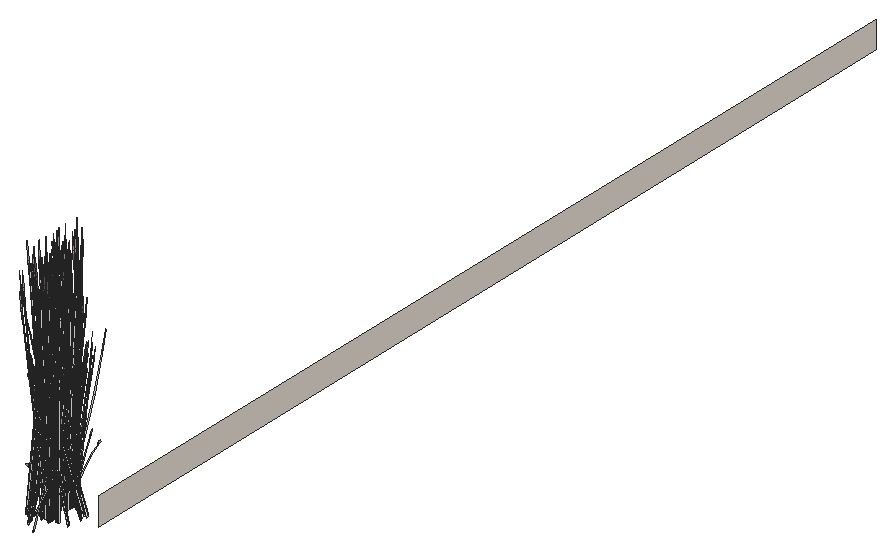
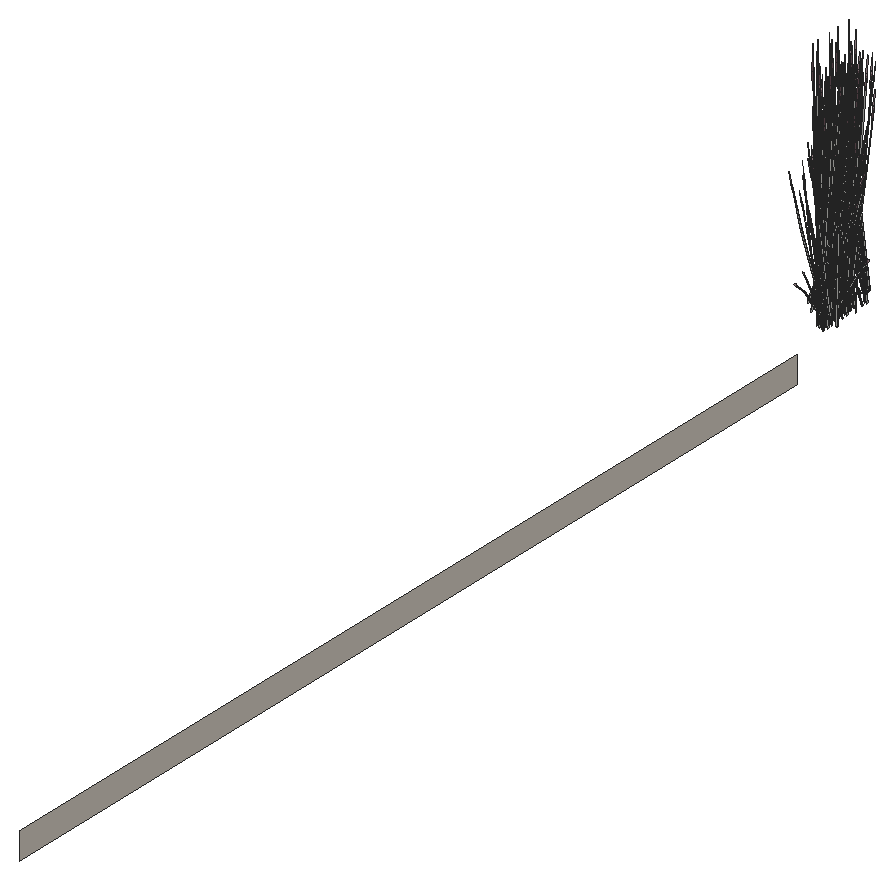
# SketchUp Ruby script. Lengths in inches.
U = 1.inch
M = Sketchup.active_model
def pt(a) = Geom::Point3d.new(a.map { |v| v * U })
def face(e, loops, mat)
  f = e.add_face(loops[0].map { |a| pt(a) })
  loops[1..].each { |l| e.add_face(l.map { |a| pt(a) }).erase! }
  f.material = f.back_material = mat if mat
  f
end
# faces: each face lists its corners as indices into pts; further lists are holes
def faces(e, pts, list, mat = nil) = list.each { |f| face(e, (f[0].is_a?(Array) ? f : [f]).map { |l| l.map { |i| pts[i] } }, mat) }
# xy, xz, yz: faces in a plane at the given z, y or x. An outline is a flat list of corners, or four numbers for a rectangle; further outlines are holes
def ring(l) = l.size == 4 ? [[l[0], l[1]], [l[2], l[1]], [l[2], l[3]], [l[0], l[3]]] : l.each_slice(2).to_a
def flat(e, list, mat, &to3) = list.each { |f| face(e, (f[0].is_a?(Array) ? f : [f]).map { |l| ring(l).map { |u, v| to3.(u, v) } }, mat) }
def xy(e, z, list, mat = nil) = flat(e, list, mat) { |x, y| [x, y, z] }
def xz(e, y, list, mat = nil) = flat(e, list, mat) { |x, z| [x, y, z] }
def yz(e, x, list, mat = nil) = flat(e, list, mat) { |y, z| [x, y, z] }
def lines(e, pts, list) = list.each { |a, b| e.add_line(pt(pts[a]), pt(pts[b])) }
# prism: a flat outline (further loops are holes) pulled along v
def prism(e, loops, v, mat = nil)
  f = face(e, loops, mat); d = Geom::Vector3d.new(v.map { |x| x * U })
  f.pushpull(f.normal.samedirection?(d) ? d.length : -d.length)
end
def box(e, o, s, mat = nil) = prism(e, [[o, [o[0] + s[0], o[1], o[2]], [o[0] + s[0], o[1] + s[1], o[2]], [o[0], o[1] + s[1], o[2]]]], [0, 0, s[2]], mat)
def at(x, y, z, deg = 0) = Geom::Transformation.translation(pt([x, y, z])) * Geom::Transformation.rotation(ORIGIN, Z_AXIS, deg.degrees)
def axes(o, x, y, z) = Geom::Transformation.new([*x, 0, *y, 0, *z, 0, *pt(o).to_a, 1])
def part(name) = M.definitions.add(name)
# library, detail: a bought-in or finely detailed component or shape, given as its bounding box
def library(name, o, s) = part(name).tap { |d| box(d.entities, o, s) }
def detail(e, o, s) = box(e.add_group.entities, o, s)
def put(e, d, t, mat = nil) = e.add_instance(d, t).tap { |i| i.material = mat if mat }
def group(e, t, mat = nil) = e.add_group.tap { |g| g.transformation = t; g.material = mat if mat }.entities
root = M.entities
M.materials.add("LightPink_Translucent").color = [144, 107, 117]
M.materials["LightPink_Translucent"].alpha = 0.75
M.materials.add("Marble_01_1K").color = [230, 221, 211]
c1 = part("blade")
p = [[2.15,0.21,22],[0,0.17,0],[0.09,0.45,0],[2.18,0.31,22],[2.29,0.31,22],[0.38,0.45,0],
  [2.48,0.24,33],[2.49,0.24,33],[2.48,0.22,33]]
faces(c1.entities,p,[[0,1,2,3],[4,5,2,3],[6,3,4,7],[8,0,3,6]])
c2 = part("seeds")
p = [[0.3,-0.1,1.38],[-0.01,-0.03,1.59],[-0.01,-0.03,0.03],[0.14,-0.07,-0.07],[0.29,-0.03,3],[0.15,0.01,3.11]]
faces(c2.entities,p,[[0,1,2,3],[1,0,4,5]],"LightPink_Translucent")
c3 = part("blade with seeds")
put(c3.entities,c1,at(0,0,0))
put(c3.entities,c2,axes([2.4,0.25,30.99],[1.5799,-0.05474,1.17369],[-0.12525,1.92788,0.29478],[-0.07173,-0.02425,1.56792]))
yz(root,314,[[46,36,262,42]],"Marble_01_1K")
put(root,c3,axes([314.17,31.27,44.36],[-0.56863,-0.18645,-0.25709],[0.2738,-0.39352,-0.44182],[-0.01787,-0.09662,1.41118]))
put(root,c3,axes([314.2,27.4,46.18],[-0.37205,0.1328,0.05682],[-0.18211,-0.24217,0.44729],[0.03593,0.10675,0.68204]))
put(root,c3,axes([313.16,26.84,46.77],[0.55492,0.01936,-0.11927],[-0.01517,0.36657,-0.66198],[-0.03855,0.14118,1.00587]))
put(root,c3,axes([314.33,27.37,46.47],[-0.49753,-0.10215,0.47081],[0.17013,-0.33585,0.3882],[0.0299,0.13207,0.97422]))
put(root,c3,axes([313.41,27.88,44.44],[-0.01307,-0.23234,1.01491],[0.32652,0.16572,0.74569],[-0.06422,0.11074,0.22354]))
put(root,c3,axes([314.27,27.32,43.32],[0.08172,-0.02126,1.55816],[0.49154,0.11703,-0.23804],[0.01437,0.1319,0.26541]))
put(root,c3,axes([313.54,26.98,46.42],[0.36145,0.26255,-0.50118],[-0.38183,0.22994,-0.3882],[-0.055,0.1334,0.95895]))
put(root,c3,axes([314.54,31.16,44.15],[0.56891,0.18939,0.21263],[-0.2738,0.39352,0.44182],[0,-0.09071,1.41855]))
put(root,c3,axes([314.31,31.6875,44.16],[0.13383,-0.46302,-0.20702],[0.63453,0.08071,0.45303],[-0.11087,-0.06394,1.38231]))
put(root,c3,axes([313.14,27.375,44.49],[0.45869,-0.0692,0.0575],[0.10545,0.27878,-0.76259],[-0.02908,0.14112,0.68355]))
put(root,c3,axes([314.38,27.44,46],[-0.15222,0.30049,-0.31292],[-0.44409,-0.08764,0.40398],[0.04072,0.12098,0.77298]))
put(root,c3,axes([314.35,30.89,44.4],[-0.54829,0.02412,0.39531],[-0.04958,-0.40041,-0.19025],[0.09816,-0.04058,1.26923]))
put(root,c3,axes([312.9375,31.18,44.19],[0,0.39075,0.43871],[-0.56491,0,0],[0,-0.089,1.3917]))
put(root,c3,axes([313.43,26.86,46.72],[-0.01314,0.36145,-0.69681],[-0.55324,-0.02428,0.08409],[-0.05838,0.15313,0.9857]))
put(root,c3,axes([314.27,31.5,43.95],[-0.30332,-0.32798,-0.39531],[0.45944,-0.23096,0.19025],[-0.09816,-0.04058,1.26923]))
put(root,c3,axes([314.33,31.04,44.09],[0.21952,0.43694,0.40429],[-0.62724,0.15194,0.15865],[0.00767,-0.08029,1.40366]))
put(root,c3,axes([313.95,26.61,45.43],[-0.01236,-0.14998,1.51428],[0.53562,0.09949,0.12244],[-0.03313,0.21373,0.64734]))
put(root,c3,axes([314.22,31.38,44.4],[-0.24498,0.3521,0.39531],[-0.50902,-0.16945,-0.19025],[0,-0.08116,1.26923]))
put(root,c3,axes([315.125,31.07,43.95],[0,-0.45213,0],[0.63136,0,0],[0,0,1.58567]))
put(root,c3,axes([314.43,27.17,46.4],[0.24099,0.31773,-0.62776],[-0.49607,0.17707,0.07576],[0.05635,0.15352,0.88802]))
put(root,c3,axes([314.07,27.98,46.17],[0.064,0.06292,1.54581],[0.51651,0.02472,-0.24447],[0.05194,0.13877,0.12397]))
put(root,c3,axes([315.28,31.42,44.03],[-0.46965,-0.33633,-0.05417],[0.46994,-0.33653,0],[-0.0164,-0.01174,1.55135]))
put(root,c3,axes([314.1,30.2,44.1875],[-0.14586,0.38834,0.15589],[-0.53375,-0.1099,0.31002],[0.0922,-0.00189,1.41735]))
put(root,c3,axes([320.46,29.24,45.43],[0.17519,-0.08265,1.51428],[0.14749,0.38193,0.12244],[-0.27504,0.08632,0.64734]))
put(root,c3,axes([314.39,31.46,44.09],[0.63817,0.08233,0.40429],[-0.12987,0.46497,0.15865],[-0.09326,-0.0449,1.40366]))
put(root,c3,axes([313.24,27.37,44.97],[0.01109,-0.20172,1.3638],[0.49896,0.10655,0.18846],[-0.04323,0.21498,0.64398]))
put(root,c3,axes([314.05,32.21,44.1875],[0.54257,-0.10371,0.15589],[0.13397,0.38597,0.31002],[-0.04839,-0.05624,1.41735]))
put(root,c3,axes([315.71,30.23,44.1875],[-0.54257,0.10371,0.15589],[-0.13397,-0.38597,0.31002],[0.04839,0.05624,1.41735]))
put(root,c3,axes([314.86,32.12,43.95],[-0.16474,-0.33688,0],[0.47043,-0.11798,0],[0,0,1.36402]))
put(root,c3,axes([314.55,31.8,44.3125],[-0.09741,0.34873,0.12794],[-0.4759,-0.06053,-0.36534],[-0.08661,-0.03581,1.11991]))
put(root,c3,axes([319.75,33.8,45.43],[0.18755,0.06732,1.51428],[-0.38813,0.28243,0.12244],[-0.24191,-0.12741,0.64734]))
put(root,c3,axes([315.66,32.23,44.1875],[0.14586,-0.38834,0.15589],[0.53375,0.1099,0.31002],[-0.0922,0.00189,1.41735]))
put(root,c3,axes([316.49,31.24,44.1875],[-0.39671,-0.28463,0.15589],[0.39978,-0.27607,0.31002],[-0.04381,0.05813,1.41735]))
put(root,c3,axes([314.74,32.27,43.94],[-0.50902,-0.17543,0],[0.24498,-0.36452,0],[0,0,1.43768]))
put(root,c3,axes([315.17,31.8,44.18],[-0.49304,-0.31451,-0.2226],[0.41487,-0.35316,0.48713],[-0.13277,0.03679,1.48635]))
put(root,c3,axes([313.87,32.4,44.19],[0.47255,0.19538,0.43871],[-0.28245,0.35034,0],[-0.10763,-0.0445,1.3917]))
put(root,c3,axes([314.27,34.43,46.17],[-0.07723,-0.05479,1.54581],[-0.51538,0.03473,-0.24447],[-0.08225,-0.13104,0.12397]))
put(root,c3,axes([314.81,35.36,46.4],[-0.24099,-0.31773,-0.62776],[0.49607,-0.17707,0.07576],[-0.05635,-0.15352,0.88802]))
put(root,c3,axes([315.44,31.25,44.03],[0,0.45191,-0.04981],[-0.63136,0,0],[0,0.0142,1.58489]))
put(root,c3,axes([314.39,34.65,43.32],[-0.08469,0.01408,1.55816],[-0.46834,-0.15847,-0.23804],[0.00786,-0.13218,0.26541]))
put(root,c3,axes([315.4,31.54,44.4],[0.54829,-0.02412,0.39531],[0.04958,0.40041,-0.19025],[-0.09816,0.04058,1.26923]))
put(root,c3,axes([314.92,31.73,43.95],[-0.54829,0.02412,-0.39531],[-0.04958,-0.40041,0.19025],[-0.09816,0.04058,1.26923]))
put(root,c3,axes([314.85,35.09,46],[0.15222,-0.30049,-0.31292],[0.44409,0.08764,0.40398],[-0.04072,-0.12098,0.77298]))
put(root,c3,axes([314.63,35.29,46.14],[-0.49634,-0.09796,-0.45151],[0.17013,-0.33585,-0.34973],[-0.04551,-0.13522,0.86392]))
put(root,c3,axes([314.93,34.45,44.44],[0.06477,0.22786,1.01491],[-0.35932,-0.1262,0.74569],[0.03867,-0.11667,0.22354]))
put(root,c3,axes([315.52,32.66,43.9375],[-0.31175,-0.39292,-0.04544],[0.52815,-0.21836,0.456],[-0.13015,0.03741,1.44584]))
put(root,c3,axes([315.41,31.71,44.3125],[0.37303,0.23477,0.12794],[-0.31115,0.26487,-0.36534],[-0.08661,0.03581,1.11991]))
put(root,c3,axes([313.64,35.08,46.5],[0.56246,-0.10044,0.47505],[0.09762,0.39398,0.3917],[-0.13228,-0.11611,0.983]))
put(root,c3,axes([314.91,35.16,46.18],[0.49753,0.10215,0.42415],[-0.17013,0.33585,0.34973],[-0.0299,-0.13207,0.87768]))
put(root,c3,axes([315.05,35.28,46.45],[-0.49409,0.18193,-0.10745],[-0.24281,-0.32289,-0.59638],[-0.06519,-0.13607,0.90619]))
put(root,c3,axes([315.8125,32.4375,44.19],[0.47255,-0.19538,0.43871],[0.28245,0.35034,0],[-0.10763,0.0445,1.3917]))
put(root,c3,axes([315.04,35.13,46.18],[0.37205,-0.1328,0.05682],[0.18211,0.24217,0.44729],[-0.03593,-0.10675,0.68204]))
put(root,c3,axes([315.14,32.13,44.02],[0.21952,0.44891,-0.05313],[-0.62724,0.1573,0],[0.00767,0.01568,1.52132]))
put(root,c3,axes([319.57,34.16,44.29],[0.09858,0.10879,1.26356],[-0.22716,0.29571,-0.27174],[-0.23325,-0.07068,0.54024]))
put(root,c3,axes([315.38,32.61,43.79],[-0.47106,-0.09668,-0.27372],[0.11861,-0.34048,0.27372],[-0.09497,0.03926,1.22797]))
put(root,c3,axes([319.98,34.0625,46.4],[-0.50473,-0.00941,-0.62776],[0.0339,-0.39618,0.07576],[-0.21383,-0.04181,0.88802]))
put(root,c3,axes([316.95,31.54,43.94],[-0.63105,-0.00312,-0.04397],[0,-0.43672,0.44129],[-0.01983,0.09942,1.3992]))
put(root,c3,axes([315.3,31.625,44.36],[0.05884,0.44587,-0.25709],[-0.6128,0.02696,-0.44182],[-0.10791,0.05939,1.41118]))
put(root,c3,axes([315.52,31.45,43.95],[-0.24498,0.3521,-0.39531],[-0.50902,-0.16945,0.19025],[0,0.08116,1.26923]))
put(root,c3,axes([313.77,35.17,46.18],[0.22948,-0.24822,0.05682],[0.32679,0.14452,0.44729],[-0.10565,-0.07958,0.68204]))
put(root,c3,axes([313.69,36.55,43.85],[-0.20736,-0.4007,-0.61707],[0.59731,-0.14431,-0.16195],[-0.02292,-0.13569,1.36206]))
put(root,c3,axes([314.9,35.4,46.46],[-0.15222,0.30049,0.31292],[-0.44409,-0.08764,-0.40398],[-0.04072,-0.12098,0.77298]))
put(root,c3,axes([315.54,32.46,44.06],[0.63212,0.12701,0.27176],[-0.15814,0.45398,-0.32244],[-0.10462,0.05682,1.45692]))
put(root,c3,axes([315.49,32.77,43.78],[-0.47255,0.19538,-0.43871],[-0.28245,-0.35034,0],[-0.10763,0.0445,1.3917]))
put(root,c3,axes([313.61,35.4,44.1],[-0.31568,-0.39156,0],[0.52815,-0.21836,-0.456],[0.12029,-0.04973,1.44655]))
put(root,c3,axes([314.31,34.92,43.88],[-0.34892,0.22417,-0.0344],[-0.3197,-0.24551,-0.15595],[-0.02251,-0.06957,0.51438]))
put(root,c3,axes([319.35,34.42,45.43],[0.20943,-0.00885,1.51428],[-0.13893,0.38357,0.12244],[-0.29846,-0.02372,0.64734]))
put(root,c3,axes([313.36,32.29,46.46],[0.34164,-0.20573,0.31292],[0.3234,0.23491,-0.40398],[-0.04921,0.11936,0.77298]))
put(root,c3,axes([315.92,32.71,44.1],[0.31568,0.39156,0],[-0.52815,0.21836,-0.456],[-0.12029,0.04973,1.44655]))
put(root,c3,axes([315.65,31.16,44.51],[-0.01379,-0.36791,1.24828],[0.62424,0.09537,0.52853],[-0.14764,0.20132,1.17828]))
put(root,c3,axes([312.47,36.49,43.78],[0,-0.39075,-0.43871],[0.56491,0,0],[0,-0.089,1.3917]))
put(root,c3,axes([314.32,32.63,46.46],[0.15222,-0.30049,0.31292],[0.44409,0.08764,-0.40398],[0.04072,0.12098,0.77298]))
put(root,c3,axes([314.01,36.65,43.95],[0.24498,-0.3521,-0.39531],[0.50902,0.16945,0.19025],[0,-0.08116,1.26923]))
put(root,c3,axes([312.71,36.5,43.79],[0.35245,-0.2438,-0.27372],[0.35245,0.2438,0.27372],[0,-0.07853,1.22797]))
put(root,c3,axes([313.95,36.94,44.36],[-0.56863,-0.18645,-0.25709],[0.2738,-0.39352,-0.44182],[-0.01787,-0.09662,1.41118]))
put(root,c3,axes([314.18,32.9,46.18],[-0.37205,0.1328,0.05682],[-0.18211,-0.24217,0.44729],[0.03593,0.10675,0.68204]))
put(root,c3,axes([313.15,32.35,46.77],[0.55492,0.01936,-0.11927],[-0.01517,0.36657,-0.66198],[-0.03855,0.14118,1.00587]))
put(root,c3,axes([314.32,32.875,46.47],[-0.49753,-0.10215,0.47081],[0.17013,-0.33585,0.3882],[0.0299,0.13207,0.97422]))
put(root,c3,axes([319.17,34.75,46],[-0.41962,-0.10901,-0.31292],[0.12239,-0.31802,0.40398],[-0.16894,0.02916,0.77298]))
put(root,c3,axes([313.4,33.38,44.44],[-0.01307,-0.23234,1.01491],[0.32652,0.16572,0.74569],[-0.06422,0.11074,0.22354]))
put(root,c3,axes([314.26,32.83,43.32],[0.08172,-0.02126,1.55816],[0.49154,0.11703,-0.23804],[0.01437,0.1319,0.26541]))
put(root,c3,axes([313.52,32.49,46.42],[0.36145,0.26255,-0.50118],[-0.38183,0.22994,-0.3882],[-0.055,0.1334,0.95895]))
put(root,c3,axes([313.13,32.88,44.49],[0.45869,-0.0692,0.0575],[0.10545,0.27878,-0.76259],[-0.02908,0.14112,0.68355]))
put(root,c3,axes([314.3125,36.83,44.15],[0.56891,0.18939,0.21263],[-0.2738,0.39352,0.44182],[0,-0.09071,1.41855]))
put(root,c3,axes([314.09,37.36,44.16],[0.13383,-0.46302,-0.20702],[0.63453,0.08071,0.45303],[-0.11087,-0.06394,1.38231]))
put(root,c3,axes([314.37,32.95,46],[-0.15222,0.30049,-0.31292],[-0.44409,-0.08764,0.40398],[0.04072,0.12098,0.77298]))
put(root,c3,axes([320.45,34.7,44.95],[0.14352,-0.05653,1.56454],[0.04949,0.39467,0.12244],[-0.31087,0.05237,0.55918]))
put(root,c3,axes([313.41,32.37,46.72],[-0.01314,0.36145,-0.69681],[-0.55324,-0.02428,0.08409],[-0.05838,0.15313,0.9857]))
put(root,c3,axes([314.13,36.5625,44.4],[-0.54829,0.02412,0.39531],[-0.04958,-0.40041,-0.19025],[0.09816,-0.04058,1.26923]))
put(root,c3,axes([313.94,32.11,45.43],[-0.01236,-0.14998,1.51428],[0.53562,0.09949,0.12244],[-0.03313,0.21373,0.64734]))
put(root,c3,axes([312.71,36.86,44.19],[0,0.39075,0.43871],[-0.56491,0,0],[0,-0.089,1.3917]))
put(root,c3,axes([314.11,36.71,44.09],[0.21952,0.43694,0.40429],[-0.62724,0.15194,0.15865],[0.00767,-0.08029,1.40366]))
put(root,c3,axes([314.42,32.68,46.4],[0.24099,0.31773,-0.62776],[-0.49607,0.17707,0.07576],[0.05635,0.15352,0.88802]))
put(root,c3,axes([318.9,34.96,46.17],[-0.08245,0.05073,1.54581],[0.00701,0.37067,-0.24447],[-0.18899,0.0482,0.12397]))
put(root,c3,axes([319.46,34.91,46.14],[-0.13679,0.35544,-0.45151],[-0.46898,-0.12183,-0.34973],[-0.18882,0.03259,0.86392]))
put(root,c3,axes([314,37.05,44.4],[-0.24498,0.3521,0.39531],[-0.50902,-0.16945,-0.19025],[0,-0.08116,1.26923]))
put(root,c3,axes([314.06,33.48,46.17],[0.064,0.06292,1.54581],[0.51651,0.02472,-0.24447],[0.05194,0.13877,0.12397]))
put(root,c3,axes([314.9,36.74,43.95],[0,-0.45213,0],[0.63136,0,0],[0,0,1.58567]))
put(root,c3,axes([314.6,36.46,44.09],[-0.41865,0.35461,0.40429],[-0.49737,-0.31303,0.15865],[0.10093,-0.03539,1.40366]))
put(root,c3,axes([315.06,37.09,44.03],[-0.46965,-0.33633,-0.05417],[0.46994,-0.33653,0],[-0.0164,-0.01174,1.55135]))
put(root,c3,axes([313.875,35.875,44.1875],[-0.14586,0.38834,0.15589],[-0.53375,-0.1099,0.31002],[0.0922,-0.00189,1.41735]))
put(root,c3,axes([313.23,32.875,44.97],[0.01109,-0.20172,1.3638],[0.49896,0.10655,0.18846],[-0.04323,0.21498,0.64398]))
put(root,c3,axes([314.17,37.14,44.09],[0.63817,0.08233,0.40429],[-0.12987,0.46497,0.15865],[-0.09326,-0.0449,1.40366]))
put(root,c3,axes([319.44,35.09,45.43],[0.17519,-0.08265,1.51428],[0.14749,0.38193,0.12244],[-0.27504,0.08632,0.64734]))
put(root,c3,axes([313.82,37.88,44.1875],[0.54257,-0.10371,0.15589],[0.13397,0.38597,0.31002],[-0.04839,-0.05624,1.41735]))
put(root,c3,axes([318.9,35.74,44.29],[0.17547,0.03208,1.26356],[0.1131,0.32764,-0.27174],[-0.23835,0.06133,0.54024]))
put(root,c3,axes([315.49,35.9,44.1875],[-0.54257,0.10371,0.15589],[-0.13397,-0.38597,0.31002],[0.04839,0.05624,1.41735]))
put(root,c3,axes([317.99,35.33,46.16],[0.06444,0.01048,1.56736],[0.19934,0.34525,-0.1481],[-0.13191,0.09062,0.27737]))
put(root,c3,axes([314.64,37.79,43.95],[-0.16474,-0.33688,0],[0.47043,-0.11798,0],[0,0,1.36402]))
put(root,c3,axes([314.32,37.47,44.3125],[-0.09741,0.34873,0.12794],[-0.4759,-0.06053,-0.36534],[-0.08661,-0.03581,1.11991]))
put(root,c3,axes([315.4375,37.9,44.1875],[0.14586,-0.38834,0.15589],[0.53375,0.1099,0.31002],[-0.0922,0.00189,1.41735]))
put(root,c3,axes([315.32,37.02,43.96],[0.35245,0.2524,0],[-0.35245,0.2524,0],[0,0,1.49564]))
put(root,c3,axes([316.27,36.91,44.1875],[-0.39671,-0.28463,0.15589],[0.39978,-0.27607,0.31002],[-0.04381,0.05813,1.41735]))
put(root,c3,axes([314.52,37.94,43.94],[-0.50902,-0.17543,0],[0.24498,-0.36452,0],[0,0,1.43768]))
put(root,c3,axes([313.65,38.08,44.19],[0.47255,0.19538,0.43871],[-0.28245,0.35034,0],[-0.10763,-0.0445,1.3917]))
put(root,c3,axes([315.3125,36.72,44.4],[0.24498,-0.3521,0.39531],[0.50902,0.16945,-0.19025],[0,0.08116,1.26923]))
put(root,c3,axes([315.22,36.93,44.03],[0,0.45191,-0.04981],[-0.63136,0,0],[0,0.0142,1.58489]))
put(root,c3,axes([315.18,37.21,44.4],[0.54829,-0.02412,0.39531],[0.04958,0.40041,-0.19025],[-0.09816,0.04058,1.26923]))
put(root,c3,axes([314.69,37.41,43.95],[-0.54829,0.02412,-0.39531],[-0.04958,-0.40041,0.19025],[-0.09816,0.04058,1.26923]))
put(root,c3,axes([315.1,37.95,43.95],[0.50902,0.17543,0],[-0.24498,0.36452,0],[0,0,1.54589]))
put(root,c3,axes([315.3,38.33,43.9375],[-0.31175,-0.39292,-0.04544],[0.52815,-0.21836,0.456],[-0.13015,0.03741,1.44584]))
put(root,c3,axes([315.19,37.38,44.3125],[0.37303,0.23477,0.12794],[-0.31115,0.26487,-0.36534],[-0.08661,0.03581,1.11991]))
put(root,c3,axes([315.59,38.11,44.19],[0.47255,-0.19538,0.43871],[0.28245,0.35034,0],[-0.10763,0.0445,1.3917]))
put(root,c3,axes([314.92,37.8,44.02],[0.21952,0.44891,-0.05313],[-0.62724,0.1573,0],[0.00767,0.01568,1.52132]))
put(root,c3,axes([315.16,38.29,43.79],[-0.47106,-0.09668,-0.27372],[0.11861,-0.34048,0.27372],[-0.09497,0.03926,1.22797]))
put(root,c3,axes([316.73,37.21,43.94],[-0.63105,-0.00312,-0.04397],[0,-0.43672,0.44129],[-0.01983,0.09942,1.3992]))
put(root,c3,axes([315.08,37.3,44.36],[0.05884,0.44587,-0.25709],[-0.6128,0.02696,-0.44182],[-0.10791,0.05939,1.41118]))
put(root,c3,axes([315.3,37.125,43.95],[-0.24498,0.3521,-0.39531],[-0.50902,-0.16945,0.19025],[0,0.08116,1.26923]))
put(root,c3,axes([315.32,38.13,44.06],[0.63212,0.12701,0.27176],[-0.15814,0.45398,-0.32244],[-0.10462,0.05682,1.45692]))
put(root,c3,axes([315.27,38.44,43.78],[-0.47255,0.19538,-0.43871],[-0.28245,-0.35034,0],[-0.10763,0.0445,1.3917]))
put(root,c3,axes([313.14,37.96,46.46],[0.34164,-0.20573,0.31292],[0.3234,0.23491,-0.40398],[-0.04921,0.11936,0.77298]))
put(root,c3,axes([315.7,38.38,44.1],[0.31568,0.39156,0],[-0.52815,0.21836,-0.456],[-0.12029,0.04973,1.44655]))
put(root,c3,axes([315.43,36.83,44.51],[-0.01379,-0.36791,1.24828],[0.62424,0.09537,0.52853],[-0.14764,0.20132,1.17828]))
put(root,c3,axes([314.1,38.3,46.46],[0.15222,-0.30049,0.31292],[0.44409,0.08764,-0.40398],[0.04072,0.12098,0.77298]))
put(root,c3,axes([314.7,39.37,46.99],[0.34892,-0.22417,-0.05733],[0.3197,0.24551,-0.25992],[0.02251,0.06957,0.85731]))
put(root,c3,axes([313.96,38.57,46.18],[-0.37205,0.1328,0.05682],[-0.18211,-0.24217,0.44729],[0.03593,0.10675,0.68204]))
put(root,c3,axes([312.92,38.02,46.77],[0.55492,0.01936,-0.11927],[-0.01517,0.36657,-0.66198],[-0.03855,0.14118,1.00587]))
put(root,c3,axes([314.09,38.55,46.47],[-0.49753,-0.10215,0.47081],[0.17013,-0.33585,0.3882],[0.0299,0.13207,0.97422]))
put(root,c3,axes([313.18,39.05,44.44],[-0.01307,-0.23234,1.01491],[0.32652,0.16572,0.74569],[-0.06422,0.11074,0.22354]))
put(root,c3,axes([314.04,38.5,43.32],[0.08172,-0.02126,1.55816],[0.49154,0.11703,-0.23804],[0.01437,0.1319,0.26541]))
put(root,c3,axes([313.3,38.16,46.42],[0.36145,0.26255,-0.50118],[-0.38183,0.22994,-0.3882],[-0.055,0.1334,0.95895]))
put(root,c3,axes([312.91,38.55,44.49],[0.45869,-0.0692,0.0575],[0.10545,0.27878,-0.76259],[-0.02908,0.14112,0.68355]))
put(root,c3,axes([314.15,38.62,46],[-0.15222,0.30049,-0.31292],[-0.44409,-0.08764,0.40398],[0.04072,0.12098,0.77298]))
put(root,c3,axes([313.71,37.78,45.43],[-0.01236,-0.14998,1.51428],[0.53562,0.09949,0.12244],[-0.03313,0.21373,0.64734]))
put(root,c3,axes([314.19,38.35,46.4],[0.24099,0.31773,-0.62776],[-0.49607,0.17707,0.07576],[0.05635,0.15352,0.88802]))
put(root,c3,axes([313.83,39.15,46.17],[0.064,0.06292,1.54581],[0.51651,0.02472,-0.24447],[0.05194,0.13877,0.12397]))
put(root,c3,axes([313,38.55,44.97],[0.01109,-0.20172,1.3638],[0.49896,0.10655,0.18846],[-0.04323,0.21498,0.64398]))
